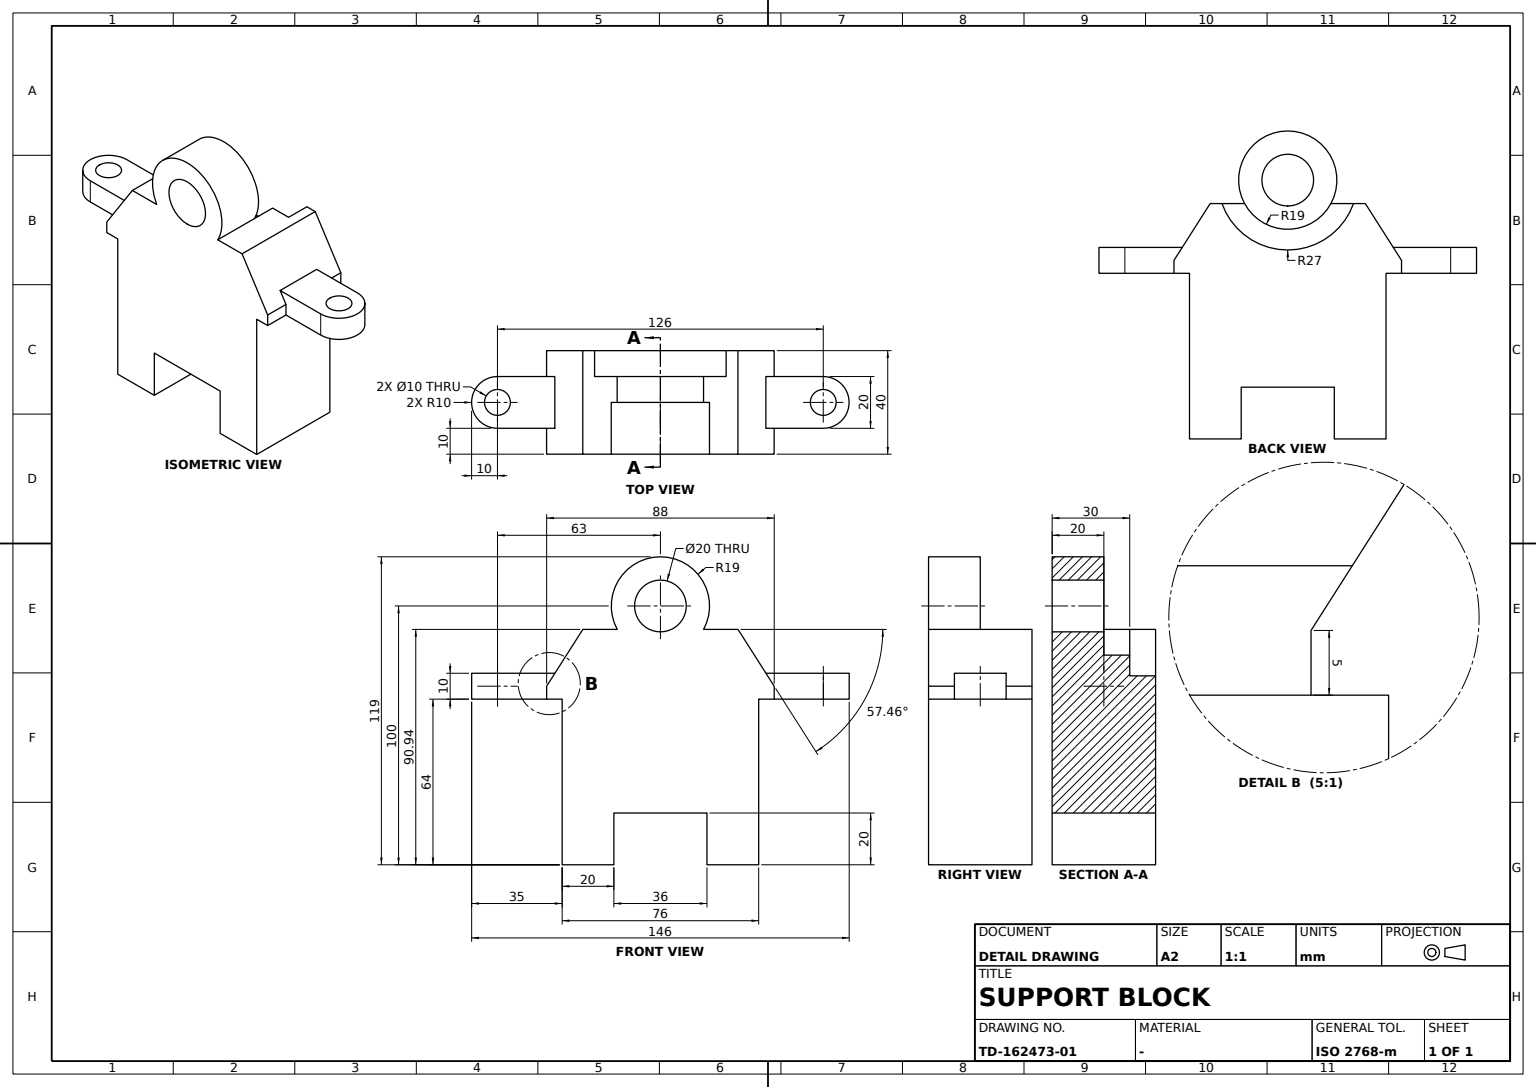
ISO-10303-21;
HEADER;
FILE_DESCRIPTION((''),'2;1');
FILE_NAME('','',(''),(''),'','','');
FILE_SCHEMA(('AUTOMOTIVE_DESIGN'));
ENDSEC;
DATA;
#1=APPLICATION_CONTEXT('');
#2=PRODUCT_CONTEXT('',#1,'mechanical');
#3=PRODUCT('','','',(#2));
#4=PRODUCT_DEFINITION_FORMATION('','',#3);
#5=PRODUCT_DEFINITION_CONTEXT('',#1,'design');
#6=PRODUCT_DEFINITION('','',#4,#5);
#7=PRODUCT_DEFINITION_SHAPE('','',#6);
#8=(LENGTH_UNIT()NAMED_UNIT(*)SI_UNIT(.MILLI.,.METRE.));
#9=(NAMED_UNIT(*)PLANE_ANGLE_UNIT()SI_UNIT($,.RADIAN.));
#10=(NAMED_UNIT(*)SI_UNIT($,.STERADIAN.)SOLID_ANGLE_UNIT());
#11=UNCERTAINTY_MEASURE_WITH_UNIT(LENGTH_MEASURE(0.005),#8,'distance_accuracy_value','');
#12=(GEOMETRIC_REPRESENTATION_CONTEXT(3)GLOBAL_UNCERTAINTY_ASSIGNED_CONTEXT((#11))GLOBAL_UNIT_ASSIGNED_CONTEXT((#8,#9,#10))REPRESENTATION_CONTEXT('',''));
#13=CARTESIAN_POINT('',(44.,10.,64.));
#14=VERTEX_POINT('',#13);
#15=CARTESIAN_POINT('',(44.,20.,64.));
#16=VERTEX_POINT('',#15);
#17=CARTESIAN_POINT('',(44.,0.,64.));
#18=DIRECTION('',(0.,1.,0.));
#19=VECTOR('',#18,1000.);
#20=LINE('',#17,#19);
#21=EDGE_CURVE('',#14,#16,#20,.T.);
#22=ORIENTED_EDGE('',*,*,#21,.T.);
#23=CARTESIAN_POINT('',(44.,20.,69.));
#24=VERTEX_POINT('',#23);
#25=CARTESIAN_POINT('',(44.,20.,0.));
#26=DIRECTION('',(0.,0.,1.));
#27=VECTOR('',#26,1000.);
#28=LINE('',#25,#27);
#29=EDGE_CURVE('',#16,#24,#28,.T.);
#30=ORIENTED_EDGE('',*,*,#29,.T.);
#31=CARTESIAN_POINT('',(44.,10.,69.));
#32=VERTEX_POINT('',#31);
#33=CARTESIAN_POINT('',(44.,0.,69.));
#34=LINE('',#33,#19);
#35=EDGE_CURVE('',#32,#24,#34,.T.);
#36=ORIENTED_EDGE('',*,*,#35,.F.);
#37=LINE('',#13,#27);
#38=EDGE_CURVE('',#14,#32,#37,.T.);
#39=ORIENTED_EDGE('',*,*,#38,.F.);
#40=EDGE_LOOP('',(#22,#30,#36,#39));
#41=FACE_BOUND('',#40,.T.);
#42=DIRECTION('',(-1.,0.,0.));
#43=AXIS2_PLACEMENT_3D('',#17,#42,#26);
#44=PLANE('',#43);
#45=ADVANCED_FACE('',(#41),#44,.F.);
#46=CARTESIAN_POINT('',(-44.,10.,64.));
#47=VERTEX_POINT('',#46);
#48=CARTESIAN_POINT('',(-44.,10.,69.));
#49=VERTEX_POINT('',#48);
#50=CARTESIAN_POINT('',(-44.,10.,0.));
#51=LINE('',#50,#27);
#52=EDGE_CURVE('',#47,#49,#51,.T.);
#53=ORIENTED_EDGE('',*,*,#52,.T.);
#54=CARTESIAN_POINT('',(-44.,20.,69.));
#55=VERTEX_POINT('',#54);
#56=CARTESIAN_POINT('',(-44.,0.,69.));
#57=LINE('',#56,#19);
#58=EDGE_CURVE('',#49,#55,#57,.T.);
#59=ORIENTED_EDGE('',*,*,#58,.T.);
#60=CARTESIAN_POINT('',(-44.,20.,64.));
#61=VERTEX_POINT('',#60);
#62=CARTESIAN_POINT('',(-44.,20.,0.));
#63=DIRECTION('',(0.,0.,-1.));
#64=VECTOR('',#63,1000.);
#65=LINE('',#62,#64);
#66=EDGE_CURVE('',#55,#61,#65,.T.);
#67=ORIENTED_EDGE('',*,*,#66,.T.);
#68=CARTESIAN_POINT('',(-44.,0.,64.));
#69=LINE('',#68,#19);
#70=EDGE_CURVE('',#47,#61,#69,.T.);
#71=ORIENTED_EDGE('',*,*,#70,.F.);
#72=EDGE_LOOP('',(#53,#59,#67,#71));
#73=FACE_BOUND('',#72,.T.);
#74=DIRECTION('',(1.,0.,0.));
#75=AXIS2_PLACEMENT_3D('',#56,#74,#63);
#76=PLANE('',#75);
#77=ADVANCED_FACE('',(#73),#76,.F.);
#78=CARTESIAN_POINT('',(-58.,0.,64.));
#79=VERTEX_POINT('',#78);
#80=CARTESIAN_POINT('',(-63.,0.,64.));
#81=AXIS2_PLACEMENT_3D('',#80,#26,#74);
#82=CIRCLE('',#81,5.);
#83=EDGE_CURVE('',#79,#79,#82,.T.);
#84=ORIENTED_EDGE('',*,*,#83,.F.);
#85=EDGE_LOOP('',(#84));
#86=FACE_BOUND('',#85,.T.);
#87=CARTESIAN_POINT('',(-68.,0.,74.));
#88=VERTEX_POINT('',#87);
#89=CARTESIAN_POINT('',(-63.,0.,74.));
#90=AXIS2_PLACEMENT_3D('',#89,#63,#42);
#91=CIRCLE('',#90,5.);
#92=EDGE_CURVE('',#88,#88,#91,.F.);
#93=ORIENTED_EDGE('',*,*,#92,.T.);
#94=EDGE_LOOP('',(#93));
#95=FACE_BOUND('',#94,.T.);
#96=CARTESIAN_POINT('',(-63.,0.,69.));
#97=AXIS2_PLACEMENT_3D('',#96,#26,#42);
#98=CYLINDRICAL_SURFACE('',#97,5.);
#99=ADVANCED_FACE('',(#86,#95),#98,.F.);
#100=CARTESIAN_POINT('',(-40.81012,10.,74.));
#101=VERTEX_POINT('',#100);
#102=DIRECTION('',(0.537842608,0.,0.843045271));
#103=VECTOR('',#102,1000.);
#104=LINE('',#48,#103);
#105=EDGE_CURVE('',#49,#101,#104,.T.);
#106=ORIENTED_EDGE('',*,*,#105,.F.);
#107=ORIENTED_EDGE('',*,*,#52,.F.);
#108=CARTESIAN_POINT('',(-63.,10.,64.));
#109=VERTEX_POINT('',#108);
#110=VECTOR('',#74,1000.);
#111=LINE('',#46,#110);
#112=EDGE_CURVE('',#109,#47,#111,.T.);
#113=ORIENTED_EDGE('',*,*,#112,.F.);
#114=CARTESIAN_POINT('',(-63.,10.,74.));
#115=VERTEX_POINT('',#114);
#116=CARTESIAN_POINT('',(-63.,10.,69.));
#117=LINE('',#116,#27);
#118=EDGE_CURVE('',#109,#115,#117,.T.);
#119=ORIENTED_EDGE('',*,*,#118,.T.);
#120=CARTESIAN_POINT('',(0.,10.,74.));
#121=LINE('',#120,#110);
#122=EDGE_CURVE('',#115,#101,#121,.T.);
#123=ORIENTED_EDGE('',*,*,#122,.T.);
#124=EDGE_LOOP('',(#106,#107,#113,#119,#123));
#125=FACE_BOUND('',#124,.T.);
#126=CARTESIAN_POINT('',(0.,10.,0.));
#127=DIRECTION('',(0.,-1.,0.));
#128=AXIS2_PLACEMENT_3D('',#126,#127,#74);
#129=PLANE('',#128);
#130=ADVANCED_FACE('',(#125),#129,.F.);
#131=CARTESIAN_POINT('',(-16.703177,-20.,90.944401));
#132=VERTEX_POINT('',#131);
#133=CARTESIAN_POINT('',(-30.,-20.,90.944401));
#134=VERTEX_POINT('',#133);
#135=CARTESIAN_POINT('',(0.,-20.,90.944401));
#136=VECTOR('',#42,1000.);
#137=LINE('',#135,#136);
#138=EDGE_CURVE('',#132,#134,#137,.T.);
#139=ORIENTED_EDGE('',*,*,#138,.T.);
#140=CARTESIAN_POINT('',(-44.,-20.,69.));
#141=VERTEX_POINT('',#140);
#142=CARTESIAN_POINT('',(-62.558286,-20.,39.910682));
#143=LINE('',#142,#103);
#144=EDGE_CURVE('',#141,#134,#143,.T.);
#145=ORIENTED_EDGE('',*,*,#144,.F.);
#146=CARTESIAN_POINT('',(-44.,-20.,64.));
#147=VERTEX_POINT('',#146);
#148=CARTESIAN_POINT('',(-44.,-20.,0.));
#149=LINE('',#148,#64);
#150=EDGE_CURVE('',#141,#147,#149,.T.);
#151=ORIENTED_EDGE('',*,*,#150,.T.);
#152=CARTESIAN_POINT('',(-38.,-20.,64.));
#153=VERTEX_POINT('',#152);
#154=CARTESIAN_POINT('',(0.,-20.,64.));
#155=LINE('',#154,#110);
#156=EDGE_CURVE('',#147,#153,#155,.T.);
#157=ORIENTED_EDGE('',*,*,#156,.T.);
#158=CARTESIAN_POINT('',(-38.,-20.,0.));
#159=VERTEX_POINT('',#158);
#160=LINE('',#158,#27);
#161=EDGE_CURVE('',#159,#153,#160,.T.);
#162=ORIENTED_EDGE('',*,*,#161,.F.);
#163=CARTESIAN_POINT('',(-18.,-20.,0.));
#164=VERTEX_POINT('',#163);
#165=CARTESIAN_POINT('',(0.,-20.,0.));
#166=LINE('',#165,#136);
#167=EDGE_CURVE('',#164,#159,#166,.T.);
#168=ORIENTED_EDGE('',*,*,#167,.F.);
#169=CARTESIAN_POINT('',(-18.,-20.,20.));
#170=VERTEX_POINT('',#169);
#171=LINE('',#163,#64);
#172=EDGE_CURVE('',#170,#164,#171,.T.);
#173=ORIENTED_EDGE('',*,*,#172,.F.);
#174=CARTESIAN_POINT('',(18.,-20.,20.));
#175=VERTEX_POINT('',#174);
#176=CARTESIAN_POINT('',(0.,-20.,20.));
#177=LINE('',#176,#136);
#178=EDGE_CURVE('',#175,#170,#177,.T.);
#179=ORIENTED_EDGE('',*,*,#178,.F.);
#180=CARTESIAN_POINT('',(18.,-20.,0.));
#181=VERTEX_POINT('',#180);
#182=LINE('',#180,#27);
#183=EDGE_CURVE('',#181,#175,#182,.T.);
#184=ORIENTED_EDGE('',*,*,#183,.F.);
#185=CARTESIAN_POINT('',(38.,-20.,0.));
#186=VERTEX_POINT('',#185);
#187=EDGE_CURVE('',#186,#181,#166,.T.);
#188=ORIENTED_EDGE('',*,*,#187,.F.);
#189=CARTESIAN_POINT('',(38.,-20.,64.));
#190=VERTEX_POINT('',#189);
#191=LINE('',#185,#64);
#192=EDGE_CURVE('',#190,#186,#191,.T.);
#193=ORIENTED_EDGE('',*,*,#192,.F.);
#194=CARTESIAN_POINT('',(44.,-20.,64.));
#195=VERTEX_POINT('',#194);
#196=EDGE_CURVE('',#190,#195,#155,.T.);
#197=ORIENTED_EDGE('',*,*,#196,.T.);
#198=CARTESIAN_POINT('',(44.,-20.,69.));
#199=VERTEX_POINT('',#198);
#200=CARTESIAN_POINT('',(44.,-20.,0.));
#201=LINE('',#200,#27);
#202=EDGE_CURVE('',#195,#199,#201,.T.);
#203=ORIENTED_EDGE('',*,*,#202,.T.);
#204=CARTESIAN_POINT('',(30.,-20.,90.944401));
#205=VERTEX_POINT('',#204);
#206=CARTESIAN_POINT('',(62.558286,-20.,39.910682));
#207=DIRECTION('',(-0.537842608,0.,0.843045271));
#208=VECTOR('',#207,1000.);
#209=LINE('',#206,#208);
#210=EDGE_CURVE('',#199,#205,#209,.T.);
#211=ORIENTED_EDGE('',*,*,#210,.T.);
#212=CARTESIAN_POINT('',(16.703177,-20.,90.944401));
#213=VERTEX_POINT('',#212);
#214=EDGE_CURVE('',#205,#213,#137,.T.);
#215=ORIENTED_EDGE('',*,*,#214,.T.);
#216=CARTESIAN_POINT('',(0.,-20.,100.));
#217=AXIS2_PLACEMENT_3D('',#216,#18,#26);
#218=CIRCLE('',#217,19.);
#219=EDGE_CURVE('',#213,#132,#218,.F.);
#220=ORIENTED_EDGE('',*,*,#219,.T.);
#221=EDGE_LOOP('',(#139,#145,#151,#157,#162,#168,#173,#179,#184,#188,#193,#197,#203,#211,#215,#220));
#222=FACE_BOUND('',#221,.T.);
#223=CARTESIAN_POINT('',(0.,-20.,110.));
#224=VERTEX_POINT('',#223);
#225=CIRCLE('',#217,10.);
#226=EDGE_CURVE('',#224,#224,#225,.F.);
#227=ORIENTED_EDGE('',*,*,#226,.F.);
#228=EDGE_LOOP('',(#227));
#229=FACE_BOUND('',#228,.T.);
#230=AXIS2_PLACEMENT_3D('',#165,#18,#42);
#231=PLANE('',#230);
#232=ADVANCED_FACE('',(#222,#229),#231,.F.);
#233=CARTESIAN_POINT('',(-44.,-10.,64.));
#234=VERTEX_POINT('',#233);
#235=CARTESIAN_POINT('',(-63.,-10.,64.));
#236=VERTEX_POINT('',#235);
#237=CARTESIAN_POINT('',(33.,-10.,64.));
#238=LINE('',#237,#136);
#239=EDGE_CURVE('',#234,#236,#238,.T.);
#240=ORIENTED_EDGE('',*,*,#239,.F.);
#241=CARTESIAN_POINT('',(-44.,-10.,69.));
#242=VERTEX_POINT('',#241);
#243=LINE('',#233,#27);
#244=EDGE_CURVE('',#234,#242,#243,.T.);
#245=ORIENTED_EDGE('',*,*,#244,.T.);
#246=CARTESIAN_POINT('',(-40.81012,-10.,74.));
#247=VERTEX_POINT('',#246);
#248=LINE('',#241,#103);
#249=EDGE_CURVE('',#242,#247,#248,.T.);
#250=ORIENTED_EDGE('',*,*,#249,.T.);
#251=CARTESIAN_POINT('',(-63.,-10.,74.));
#252=VERTEX_POINT('',#251);
#253=CARTESIAN_POINT('',(0.,-10.,74.));
#254=LINE('',#253,#136);
#255=EDGE_CURVE('',#247,#252,#254,.T.);
#256=ORIENTED_EDGE('',*,*,#255,.T.);
#257=CARTESIAN_POINT('',(-63.,-10.,69.));
#258=LINE('',#257,#27);
#259=EDGE_CURVE('',#236,#252,#258,.T.);
#260=ORIENTED_EDGE('',*,*,#259,.F.);
#261=EDGE_LOOP('',(#240,#245,#250,#256,#260));
#262=FACE_BOUND('',#261,.T.);
#263=AXIS2_PLACEMENT_3D('',#237,#127,#74);
#264=PLANE('',#263);
#265=ADVANCED_FACE('',(#262),#264,.T.);
#266=ORIENTED_EDGE('',*,*,#219,.F.);
#267=CARTESIAN_POINT('',(16.703177,0.,90.944401));
#268=VERTEX_POINT('',#267);
#269=VECTOR('',#127,1000.);
#270=LINE('',#212,#269);
#271=EDGE_CURVE('',#213,#268,#270,.F.);
#272=ORIENTED_EDGE('',*,*,#271,.T.);
#273=CARTESIAN_POINT('',(-16.703177,0.,90.944401));
#274=VERTEX_POINT('',#273);
#275=CARTESIAN_POINT('',(0.,0.,100.));
#276=AXIS2_PLACEMENT_3D('',#275,#127,#63);
#277=CIRCLE('',#276,19.);
#278=EDGE_CURVE('',#268,#274,#277,.T.);
#279=ORIENTED_EDGE('',*,*,#278,.T.);
#280=LINE('',#131,#269);
#281=EDGE_CURVE('',#132,#274,#280,.F.);
#282=ORIENTED_EDGE('',*,*,#281,.F.);
#283=EDGE_LOOP('',(#266,#272,#279,#282));
#284=FACE_BOUND('',#283,.T.);
#285=CARTESIAN_POINT('',(0.,-10.,100.));
#286=AXIS2_PLACEMENT_3D('',#285,#127,#74);
#287=CYLINDRICAL_SURFACE('',#286,19.);
#288=ADVANCED_FACE('',(#284),#287,.T.);
#289=ORIENTED_EDGE('',*,*,#226,.T.);
#290=EDGE_LOOP('',(#289));
#291=FACE_BOUND('',#290,.T.);
#292=CARTESIAN_POINT('',(0.,0.,90.));
#293=VERTEX_POINT('',#292);
#294=CIRCLE('',#276,10.);
#295=EDGE_CURVE('',#293,#293,#294,.T.);
#296=ORIENTED_EDGE('',*,*,#295,.F.);
#297=EDGE_LOOP('',(#296));
#298=FACE_BOUND('',#297,.T.);
#299=CYLINDRICAL_SURFACE('',#286,10.);
#300=ADVANCED_FACE('',(#291,#298),#299,.F.);
#301=CARTESIAN_POINT('',(58.,0.,74.));
#302=VERTEX_POINT('',#301);
#303=CARTESIAN_POINT('',(63.,0.,74.));
#304=AXIS2_PLACEMENT_3D('',#303,#63,#42);
#305=CIRCLE('',#304,5.);
#306=EDGE_CURVE('',#302,#302,#305,.T.);
#307=ORIENTED_EDGE('',*,*,#306,.F.);
#308=EDGE_LOOP('',(#307));
#309=FACE_BOUND('',#308,.T.);
#310=CARTESIAN_POINT('',(68.,0.,64.));
#311=VERTEX_POINT('',#310);
#312=CARTESIAN_POINT('',(63.,0.,64.));
#313=AXIS2_PLACEMENT_3D('',#312,#26,#74);
#314=CIRCLE('',#313,5.);
#315=EDGE_CURVE('',#311,#311,#314,.F.);
#316=ORIENTED_EDGE('',*,*,#315,.T.);
#317=EDGE_LOOP('',(#316));
#318=FACE_BOUND('',#317,.T.);
#319=CARTESIAN_POINT('',(63.,0.,69.));
#320=AXIS2_PLACEMENT_3D('',#319,#63,#74);
#321=CYLINDRICAL_SURFACE('',#320,5.);
#322=ADVANCED_FACE('',(#309,#318),#321,.F.);
#323=CARTESIAN_POINT('',(38.,20.,0.));
#324=VERTEX_POINT('',#323);
#325=CARTESIAN_POINT('',(38.,0.,0.));
#326=LINE('',#325,#19);
#327=EDGE_CURVE('',#186,#324,#326,.T.);
#328=ORIENTED_EDGE('',*,*,#327,.F.);
#329=ORIENTED_EDGE('',*,*,#187,.T.);
#330=CARTESIAN_POINT('',(18.,20.,0.));
#331=VERTEX_POINT('',#330);
#332=CARTESIAN_POINT('',(18.,0.,0.));
#333=LINE('',#332,#19);
#334=EDGE_CURVE('',#181,#331,#333,.T.);
#335=ORIENTED_EDGE('',*,*,#334,.T.);
#336=CARTESIAN_POINT('',(0.,20.,0.));
#337=LINE('',#336,#136);
#338=EDGE_CURVE('',#324,#331,#337,.T.);
#339=ORIENTED_EDGE('',*,*,#338,.F.);
#340=EDGE_LOOP('',(#328,#329,#335,#339));
#341=FACE_BOUND('',#340,.T.);
#342=AXIS2_PLACEMENT_3D('',#325,#63,#42);
#343=PLANE('',#342);
#344=ADVANCED_FACE('',(#341),#343,.T.);
#345=EDGE_CURVE('',#147,#234,#69,.T.);
#346=ORIENTED_EDGE('',*,*,#345,.F.);
#347=ORIENTED_EDGE('',*,*,#150,.F.);
#348=EDGE_CURVE('',#141,#242,#57,.T.);
#349=ORIENTED_EDGE('',*,*,#348,.T.);
#350=ORIENTED_EDGE('',*,*,#244,.F.);
#351=EDGE_LOOP('',(#346,#347,#349,#350));
#352=FACE_BOUND('',#351,.T.);
#353=ADVANCED_FACE('',(#352),#76,.F.);
#354=CARTESIAN_POINT('',(25.436118,20.,90.944401));
#355=VERTEX_POINT('',#354);
#356=CARTESIAN_POINT('',(-25.436118,20.,90.944401));
#357=VERTEX_POINT('',#356);
#358=CARTESIAN_POINT('',(0.,20.,100.));
#359=AXIS2_PLACEMENT_3D('',#358,#18,#26);
#360=CIRCLE('',#359,27.);
#361=EDGE_CURVE('',#355,#357,#360,.T.);
#362=ORIENTED_EDGE('',*,*,#361,.T.);
#363=CARTESIAN_POINT('',(-25.436118,10.,90.944401));
#364=VERTEX_POINT('',#363);
#365=LINE('',#363,#19);
#366=EDGE_CURVE('',#364,#357,#365,.T.);
#367=ORIENTED_EDGE('',*,*,#366,.F.);
#368=CARTESIAN_POINT('',(25.436118,10.,90.944401));
#369=VERTEX_POINT('',#368);
#370=CARTESIAN_POINT('',(0.,10.,100.));
#371=AXIS2_PLACEMENT_3D('',#370,#127,#63);
#372=CIRCLE('',#371,27.);
#373=EDGE_CURVE('',#364,#369,#372,.T.);
#374=ORIENTED_EDGE('',*,*,#373,.T.);
#375=LINE('',#368,#19);
#376=EDGE_CURVE('',#369,#355,#375,.T.);
#377=ORIENTED_EDGE('',*,*,#376,.T.);
#378=EDGE_LOOP('',(#362,#367,#374,#377));
#379=FACE_BOUND('',#378,.T.);
#380=AXIS2_PLACEMENT_3D('',#275,#18,#42);
#381=CYLINDRICAL_SURFACE('',#380,27.);
#382=ADVANCED_FACE('',(#379),#381,.F.);
#383=CIRCLE('',#81,10.);
#384=EDGE_CURVE('',#109,#236,#383,.T.);
#385=ORIENTED_EDGE('',*,*,#384,.T.);
#386=ORIENTED_EDGE('',*,*,#259,.T.);
#387=CIRCLE('',#90,10.);
#388=EDGE_CURVE('',#115,#252,#387,.F.);
#389=ORIENTED_EDGE('',*,*,#388,.F.);
#390=ORIENTED_EDGE('',*,*,#118,.F.);
#391=EDGE_LOOP('',(#385,#386,#389,#390));
#392=FACE_BOUND('',#391,.T.);
#393=CYLINDRICAL_SURFACE('',#97,10.);
#394=ADVANCED_FACE('',(#392),#393,.T.);
#395=CARTESIAN_POINT('',(-30.,20.,90.944401));
#396=VERTEX_POINT('',#395);
#397=CARTESIAN_POINT('',(0.,20.,90.944401));
#398=LINE('',#397,#136);
#399=EDGE_CURVE('',#357,#396,#398,.T.);
#400=ORIENTED_EDGE('',*,*,#399,.T.);
#401=CARTESIAN_POINT('',(-30.,0.,90.944401));
#402=LINE('',#401,#19);
#403=EDGE_CURVE('',#134,#396,#402,.T.);
#404=ORIENTED_EDGE('',*,*,#403,.F.);
#405=ORIENTED_EDGE('',*,*,#138,.F.);
#406=ORIENTED_EDGE('',*,*,#281,.T.);
#407=CARTESIAN_POINT('',(-16.703177,10.,90.944401));
#408=VERTEX_POINT('',#407);
#409=LINE('',#273,#269);
#410=EDGE_CURVE('',#274,#408,#409,.F.);
#411=ORIENTED_EDGE('',*,*,#410,.T.);
#412=CARTESIAN_POINT('',(0.,10.,90.944401));
#413=LINE('',#412,#110);
#414=EDGE_CURVE('',#364,#408,#413,.T.);
#415=ORIENTED_EDGE('',*,*,#414,.F.);
#416=ORIENTED_EDGE('',*,*,#366,.T.);
#417=EDGE_LOOP('',(#400,#404,#405,#406,#411,#415,#416));
#418=FACE_BOUND('',#417,.T.);
#419=CARTESIAN_POINT('',(-25.436118,0.,90.944401));
#420=AXIS2_PLACEMENT_3D('',#419,#63,#42);
#421=PLANE('',#420);
#422=ADVANCED_FACE('',(#418),#421,.F.);
#423=CARTESIAN_POINT('',(16.703177,10.,90.944401));
#424=VERTEX_POINT('',#423);
#425=CIRCLE('',#371,19.);
#426=EDGE_CURVE('',#408,#424,#425,.T.);
#427=ORIENTED_EDGE('',*,*,#426,.T.);
#428=EDGE_CURVE('',#424,#369,#413,.T.);
#429=ORIENTED_EDGE('',*,*,#428,.T.);
#430=ORIENTED_EDGE('',*,*,#373,.F.);
#431=ORIENTED_EDGE('',*,*,#414,.T.);
#432=EDGE_LOOP('',(#427,#429,#430,#431));
#433=FACE_BOUND('',#432,.T.);
#434=ADVANCED_FACE('',(#433),#129,.F.);
#435=CARTESIAN_POINT('',(18.,20.,20.));
#436=VERTEX_POINT('',#435);
#437=LINE('',#330,#27);
#438=EDGE_CURVE('',#331,#436,#437,.T.);
#439=ORIENTED_EDGE('',*,*,#438,.F.);
#440=ORIENTED_EDGE('',*,*,#334,.F.);
#441=ORIENTED_EDGE('',*,*,#183,.T.);
#442=CARTESIAN_POINT('',(18.,0.,20.));
#443=LINE('',#442,#19);
#444=EDGE_CURVE('',#175,#436,#443,.T.);
#445=ORIENTED_EDGE('',*,*,#444,.T.);
#446=EDGE_LOOP('',(#439,#440,#441,#445));
#447=FACE_BOUND('',#446,.T.);
#448=AXIS2_PLACEMENT_3D('',#332,#42,#26);
#449=PLANE('',#448);
#450=ADVANCED_FACE('',(#447),#449,.T.);
#451=ORIENTED_EDGE('',*,*,#172,.T.);
#452=CARTESIAN_POINT('',(-18.,20.,0.));
#453=VERTEX_POINT('',#452);
#454=CARTESIAN_POINT('',(-18.,0.,0.));
#455=LINE('',#454,#19);
#456=EDGE_CURVE('',#164,#453,#455,.T.);
#457=ORIENTED_EDGE('',*,*,#456,.T.);
#458=CARTESIAN_POINT('',(-18.,20.,20.));
#459=VERTEX_POINT('',#458);
#460=LINE('',#452,#64);
#461=EDGE_CURVE('',#459,#453,#460,.T.);
#462=ORIENTED_EDGE('',*,*,#461,.F.);
#463=CARTESIAN_POINT('',(-18.,0.,20.));
#464=LINE('',#463,#19);
#465=EDGE_CURVE('',#170,#459,#464,.T.);
#466=ORIENTED_EDGE('',*,*,#465,.F.);
#467=EDGE_LOOP('',(#451,#457,#462,#466));
#468=FACE_BOUND('',#467,.T.);
#469=AXIS2_PLACEMENT_3D('',#463,#74,#63);
#470=PLANE('',#469);
#471=ADVANCED_FACE('',(#468),#470,.T.);
#472=ORIENTED_EDGE('',*,*,#426,.F.);
#473=ORIENTED_EDGE('',*,*,#410,.F.);
#474=EDGE_CURVE('',#274,#268,#277,.T.);
#475=ORIENTED_EDGE('',*,*,#474,.T.);
#476=LINE('',#267,#269);
#477=EDGE_CURVE('',#268,#424,#476,.F.);
#478=ORIENTED_EDGE('',*,*,#477,.T.);
#479=EDGE_LOOP('',(#472,#473,#475,#478));
#480=FACE_BOUND('',#479,.T.);
#481=ADVANCED_FACE('',(#480),#287,.F.);
#482=ORIENTED_EDGE('',*,*,#92,.F.);
#483=EDGE_LOOP('',(#482));
#484=FACE_BOUND('',#483,.T.);
#485=ORIENTED_EDGE('',*,*,#388,.T.);
#486=ORIENTED_EDGE('',*,*,#255,.F.);
#487=CARTESIAN_POINT('',(-40.81012,0.,74.));
#488=LINE('',#487,#19);
#489=EDGE_CURVE('',#247,#101,#488,.T.);
#490=ORIENTED_EDGE('',*,*,#489,.T.);
#491=ORIENTED_EDGE('',*,*,#122,.F.);
#492=EDGE_LOOP('',(#485,#486,#490,#491));
#493=FACE_BOUND('',#492,.T.);
#494=CARTESIAN_POINT('',(0.,0.,74.));
#495=AXIS2_PLACEMENT_3D('',#494,#63,#74);
#496=PLANE('',#495);
#497=ADVANCED_FACE('',(#484,#493),#496,.F.);
#498=ORIENTED_EDGE('',*,*,#456,.F.);
#499=ORIENTED_EDGE('',*,*,#167,.T.);
#500=CARTESIAN_POINT('',(-38.,20.,0.));
#501=VERTEX_POINT('',#500);
#502=CARTESIAN_POINT('',(-38.,0.,0.));
#503=LINE('',#502,#19);
#504=EDGE_CURVE('',#159,#501,#503,.T.);
#505=ORIENTED_EDGE('',*,*,#504,.T.);
#506=EDGE_CURVE('',#453,#501,#337,.T.);
#507=ORIENTED_EDGE('',*,*,#506,.F.);
#508=EDGE_LOOP('',(#498,#499,#505,#507));
#509=FACE_BOUND('',#508,.T.);
#510=ADVANCED_FACE('',(#509),#343,.T.);
#511=CARTESIAN_POINT('',(44.,-10.,69.));
#512=VERTEX_POINT('',#511);
#513=CARTESIAN_POINT('',(40.81012,-10.,74.));
#514=VERTEX_POINT('',#513);
#515=LINE('',#511,#208);
#516=EDGE_CURVE('',#512,#514,#515,.T.);
#517=ORIENTED_EDGE('',*,*,#516,.F.);
#518=CARTESIAN_POINT('',(44.,-10.,64.));
#519=VERTEX_POINT('',#518);
#520=LINE('',#518,#27);
#521=EDGE_CURVE('',#519,#512,#520,.T.);
#522=ORIENTED_EDGE('',*,*,#521,.F.);
#523=CARTESIAN_POINT('',(63.,-10.,64.));
#524=VERTEX_POINT('',#523);
#525=LINE('',#233,#110);
#526=EDGE_CURVE('',#519,#524,#525,.T.);
#527=ORIENTED_EDGE('',*,*,#526,.T.);
#528=CARTESIAN_POINT('',(63.,-10.,74.));
#529=VERTEX_POINT('',#528);
#530=CARTESIAN_POINT('',(63.,-10.,69.));
#531=LINE('',#530,#64);
#532=EDGE_CURVE('',#524,#529,#531,.F.);
#533=ORIENTED_EDGE('',*,*,#532,.T.);
#534=CARTESIAN_POINT('',(33.,-10.,74.));
#535=LINE('',#534,#110);
#536=EDGE_CURVE('',#514,#529,#535,.T.);
#537=ORIENTED_EDGE('',*,*,#536,.F.);
#538=EDGE_LOOP('',(#517,#522,#527,#533,#537));
#539=FACE_BOUND('',#538,.T.);
#540=ADVANCED_FACE('',(#539),#264,.T.);
#541=ORIENTED_EDGE('',*,*,#521,.T.);
#542=EDGE_CURVE('',#199,#512,#34,.T.);
#543=ORIENTED_EDGE('',*,*,#542,.F.);
#544=ORIENTED_EDGE('',*,*,#202,.F.);
#545=EDGE_CURVE('',#195,#519,#20,.T.);
#546=ORIENTED_EDGE('',*,*,#545,.T.);
#547=EDGE_LOOP('',(#541,#543,#544,#546));
#548=FACE_BOUND('',#547,.T.);
#549=ADVANCED_FACE('',(#548),#44,.F.);
#550=CARTESIAN_POINT('',(30.,20.,90.944401));
#551=VERTEX_POINT('',#550);
#552=EDGE_CURVE('',#551,#355,#398,.T.);
#553=ORIENTED_EDGE('',*,*,#552,.T.);
#554=ORIENTED_EDGE('',*,*,#376,.F.);
#555=ORIENTED_EDGE('',*,*,#428,.F.);
#556=ORIENTED_EDGE('',*,*,#477,.F.);
#557=ORIENTED_EDGE('',*,*,#271,.F.);
#558=ORIENTED_EDGE('',*,*,#214,.F.);
#559=CARTESIAN_POINT('',(30.,0.,90.944401));
#560=LINE('',#559,#19);
#561=EDGE_CURVE('',#205,#551,#560,.T.);
#562=ORIENTED_EDGE('',*,*,#561,.T.);
#563=EDGE_LOOP('',(#553,#554,#555,#556,#557,#558,#562));
#564=FACE_BOUND('',#563,.T.);
#565=ADVANCED_FACE('',(#564),#421,.F.);
#566=ORIENTED_EDGE('',*,*,#444,.F.);
#567=ORIENTED_EDGE('',*,*,#178,.T.);
#568=ORIENTED_EDGE('',*,*,#465,.T.);
#569=CARTESIAN_POINT('',(0.,20.,20.));
#570=LINE('',#569,#136);
#571=EDGE_CURVE('',#436,#459,#570,.T.);
#572=ORIENTED_EDGE('',*,*,#571,.F.);
#573=EDGE_LOOP('',(#566,#567,#568,#572));
#574=FACE_BOUND('',#573,.T.);
#575=AXIS2_PLACEMENT_3D('',#442,#63,#42);
#576=PLANE('',#575);
#577=ADVANCED_FACE('',(#574),#576,.T.);
#578=CARTESIAN_POINT('',(63.,10.,74.));
#579=VERTEX_POINT('',#578);
#580=CIRCLE('',#304,10.);
#581=EDGE_CURVE('',#579,#529,#580,.T.);
#582=ORIENTED_EDGE('',*,*,#581,.T.);
#583=ORIENTED_EDGE('',*,*,#532,.F.);
#584=CARTESIAN_POINT('',(63.,10.,64.));
#585=VERTEX_POINT('',#584);
#586=CIRCLE('',#313,10.);
#587=EDGE_CURVE('',#585,#524,#586,.F.);
#588=ORIENTED_EDGE('',*,*,#587,.F.);
#589=CARTESIAN_POINT('',(63.,10.,69.));
#590=LINE('',#589,#64);
#591=EDGE_CURVE('',#585,#579,#590,.F.);
#592=ORIENTED_EDGE('',*,*,#591,.T.);
#593=EDGE_LOOP('',(#582,#583,#588,#592));
#594=FACE_BOUND('',#593,.T.);
#595=CYLINDRICAL_SURFACE('',#320,10.);
#596=ADVANCED_FACE('',(#594),#595,.T.);
#597=CARTESIAN_POINT('',(38.,20.,64.));
#598=VERTEX_POINT('',#597);
#599=LINE('',#323,#64);
#600=EDGE_CURVE('',#598,#324,#599,.T.);
#601=ORIENTED_EDGE('',*,*,#600,.F.);
#602=CARTESIAN_POINT('',(38.,0.,64.));
#603=LINE('',#602,#19);
#604=EDGE_CURVE('',#190,#598,#603,.T.);
#605=ORIENTED_EDGE('',*,*,#604,.F.);
#606=ORIENTED_EDGE('',*,*,#192,.T.);
#607=ORIENTED_EDGE('',*,*,#327,.T.);
#608=EDGE_LOOP('',(#601,#605,#606,#607));
#609=FACE_BOUND('',#608,.T.);
#610=AXIS2_PLACEMENT_3D('',#602,#74,#63);
#611=PLANE('',#610);
#612=ADVANCED_FACE('',(#609),#611,.T.);
#613=ORIENTED_EDGE('',*,*,#438,.T.);
#614=ORIENTED_EDGE('',*,*,#571,.T.);
#615=ORIENTED_EDGE('',*,*,#461,.T.);
#616=ORIENTED_EDGE('',*,*,#506,.T.);
#617=CARTESIAN_POINT('',(-38.,20.,64.));
#618=VERTEX_POINT('',#617);
#619=LINE('',#500,#27);
#620=EDGE_CURVE('',#501,#618,#619,.T.);
#621=ORIENTED_EDGE('',*,*,#620,.T.);
#622=CARTESIAN_POINT('',(0.,20.,64.));
#623=LINE('',#622,#110);
#624=EDGE_CURVE('',#61,#618,#623,.T.);
#625=ORIENTED_EDGE('',*,*,#624,.F.);
#626=ORIENTED_EDGE('',*,*,#66,.F.);
#627=CARTESIAN_POINT('',(-62.558286,20.,39.910682));
#628=LINE('',#627,#103);
#629=EDGE_CURVE('',#55,#396,#628,.T.);
#630=ORIENTED_EDGE('',*,*,#629,.T.);
#631=ORIENTED_EDGE('',*,*,#399,.F.);
#632=ORIENTED_EDGE('',*,*,#361,.F.);
#633=ORIENTED_EDGE('',*,*,#552,.F.);
#634=CARTESIAN_POINT('',(62.558286,20.,39.910682));
#635=LINE('',#634,#208);
#636=EDGE_CURVE('',#24,#551,#635,.T.);
#637=ORIENTED_EDGE('',*,*,#636,.F.);
#638=ORIENTED_EDGE('',*,*,#29,.F.);
#639=EDGE_CURVE('',#598,#16,#623,.T.);
#640=ORIENTED_EDGE('',*,*,#639,.F.);
#641=ORIENTED_EDGE('',*,*,#600,.T.);
#642=ORIENTED_EDGE('',*,*,#338,.T.);
#643=EDGE_LOOP('',(#613,#614,#615,#616,#621,#625,#626,#630,#631,#632,#633,#637,#638,#640,#641,#642));
#644=FACE_BOUND('',#643,.T.);
#645=AXIS2_PLACEMENT_3D('',#336,#18,#42);
#646=PLANE('',#645);
#647=ADVANCED_FACE('',(#644),#646,.T.);
#648=CARTESIAN_POINT('',(-38.,0.,64.));
#649=LINE('',#648,#19);
#650=EDGE_CURVE('',#153,#618,#649,.T.);
#651=ORIENTED_EDGE('',*,*,#650,.T.);
#652=ORIENTED_EDGE('',*,*,#620,.F.);
#653=ORIENTED_EDGE('',*,*,#504,.F.);
#654=ORIENTED_EDGE('',*,*,#161,.T.);
#655=EDGE_LOOP('',(#651,#652,#653,#654));
#656=FACE_BOUND('',#655,.T.);
#657=AXIS2_PLACEMENT_3D('',#502,#42,#26);
#658=PLANE('',#657);
#659=ADVANCED_FACE('',(#656),#658,.T.);
#660=ORIENTED_EDGE('',*,*,#210,.F.);
#661=ORIENTED_EDGE('',*,*,#542,.T.);
#662=ORIENTED_EDGE('',*,*,#516,.T.);
#663=CARTESIAN_POINT('',(40.81012,10.,74.));
#664=VERTEX_POINT('',#663);
#665=CARTESIAN_POINT('',(40.81012,0.,74.));
#666=LINE('',#665,#19);
#667=EDGE_CURVE('',#514,#664,#666,.T.);
#668=ORIENTED_EDGE('',*,*,#667,.T.);
#669=LINE('',#31,#208);
#670=EDGE_CURVE('',#32,#664,#669,.T.);
#671=ORIENTED_EDGE('',*,*,#670,.F.);
#672=ORIENTED_EDGE('',*,*,#35,.T.);
#673=ORIENTED_EDGE('',*,*,#636,.T.);
#674=ORIENTED_EDGE('',*,*,#561,.F.);
#675=EDGE_LOOP('',(#660,#661,#662,#668,#671,#672,#673,#674));
#676=FACE_BOUND('',#675,.T.);
#677=DIRECTION('',(-0.843045271,0.,-0.537842608));
#678=AXIS2_PLACEMENT_3D('',#33,#677,#207);
#679=PLANE('',#678);
#680=ADVANCED_FACE('',(#676),#679,.F.);
#681=ORIENTED_EDGE('',*,*,#474,.F.);
#682=ORIENTED_EDGE('',*,*,#278,.F.);
#683=EDGE_LOOP('',(#681,#682));
#684=FACE_BOUND('',#683,.T.);
#685=ORIENTED_EDGE('',*,*,#295,.T.);
#686=EDGE_LOOP('',(#685));
#687=FACE_BOUND('',#686,.T.);
#688=CARTESIAN_POINT('',(0.,0.,0.));
#689=AXIS2_PLACEMENT_3D('',#688,#127,#74);
#690=PLANE('',#689);
#691=ADVANCED_FACE('',(#684,#687),#690,.F.);
#692=ORIENTED_EDGE('',*,*,#639,.T.);
#693=ORIENTED_EDGE('',*,*,#21,.F.);
#694=CARTESIAN_POINT('',(0.,10.,64.));
#695=LINE('',#694,#136);
#696=EDGE_CURVE('',#585,#14,#695,.T.);
#697=ORIENTED_EDGE('',*,*,#696,.F.);
#698=ORIENTED_EDGE('',*,*,#587,.T.);
#699=ORIENTED_EDGE('',*,*,#526,.F.);
#700=ORIENTED_EDGE('',*,*,#545,.F.);
#701=ORIENTED_EDGE('',*,*,#196,.F.);
#702=ORIENTED_EDGE('',*,*,#604,.T.);
#703=EDGE_LOOP('',(#692,#693,#697,#698,#699,#700,#701,#702));
#704=FACE_BOUND('',#703,.T.);
#705=ORIENTED_EDGE('',*,*,#315,.F.);
#706=EDGE_LOOP('',(#705));
#707=FACE_BOUND('',#706,.T.);
#708=AXIS2_PLACEMENT_3D('',#68,#26,#74);
#709=PLANE('',#708);
#710=ADVANCED_FACE('',(#704,#707),#709,.F.);
#711=ORIENTED_EDGE('',*,*,#591,.F.);
#712=ORIENTED_EDGE('',*,*,#696,.T.);
#713=ORIENTED_EDGE('',*,*,#38,.T.);
#714=ORIENTED_EDGE('',*,*,#670,.T.);
#715=LINE('',#120,#136);
#716=EDGE_CURVE('',#579,#664,#715,.T.);
#717=ORIENTED_EDGE('',*,*,#716,.F.);
#718=EDGE_LOOP('',(#711,#712,#713,#714,#717));
#719=FACE_BOUND('',#718,.T.);
#720=ADVANCED_FACE('',(#719),#129,.F.);
#721=ORIENTED_EDGE('',*,*,#144,.T.);
#722=ORIENTED_EDGE('',*,*,#403,.T.);
#723=ORIENTED_EDGE('',*,*,#629,.F.);
#724=ORIENTED_EDGE('',*,*,#58,.F.);
#725=ORIENTED_EDGE('',*,*,#105,.T.);
#726=ORIENTED_EDGE('',*,*,#489,.F.);
#727=ORIENTED_EDGE('',*,*,#249,.F.);
#728=ORIENTED_EDGE('',*,*,#348,.F.);
#729=EDGE_LOOP('',(#721,#722,#723,#724,#725,#726,#727,#728));
#730=FACE_BOUND('',#729,.T.);
#731=DIRECTION('',(-0.843045271,0.,0.537842608));
#732=AXIS2_PLACEMENT_3D('',#56,#731,#102);
#733=PLANE('',#732);
#734=ADVANCED_FACE('',(#730),#733,.T.);
#735=ORIENTED_EDGE('',*,*,#83,.T.);
#736=EDGE_LOOP('',(#735));
#737=FACE_BOUND('',#736,.T.);
#738=ORIENTED_EDGE('',*,*,#239,.T.);
#739=ORIENTED_EDGE('',*,*,#384,.F.);
#740=ORIENTED_EDGE('',*,*,#112,.T.);
#741=ORIENTED_EDGE('',*,*,#70,.T.);
#742=ORIENTED_EDGE('',*,*,#624,.T.);
#743=ORIENTED_EDGE('',*,*,#650,.F.);
#744=ORIENTED_EDGE('',*,*,#156,.F.);
#745=ORIENTED_EDGE('',*,*,#345,.T.);
#746=EDGE_LOOP('',(#738,#739,#740,#741,#742,#743,#744,#745));
#747=FACE_BOUND('',#746,.T.);
#748=ADVANCED_FACE('',(#737,#747),#709,.F.);
#749=ORIENTED_EDGE('',*,*,#306,.T.);
#750=EDGE_LOOP('',(#749));
#751=FACE_BOUND('',#750,.T.);
#752=ORIENTED_EDGE('',*,*,#667,.F.);
#753=ORIENTED_EDGE('',*,*,#536,.T.);
#754=ORIENTED_EDGE('',*,*,#581,.F.);
#755=ORIENTED_EDGE('',*,*,#716,.T.);
#756=EDGE_LOOP('',(#752,#753,#754,#755));
#757=FACE_BOUND('',#756,.T.);
#758=ADVANCED_FACE('',(#751,#757),#496,.F.);
#759=CLOSED_SHELL('',(#45,#77,#99,#130,#232,#265,#288,#300,#322,#344,#353,#382,#394,#422,#434,#450,#471,#481,#497,#510,#540,#549,#565,#577,#596,#612,#647,#659,#680,#691,#710,#720,#734,#748,#758));
#760=MANIFOLD_SOLID_BREP('',#759);
#761=ADVANCED_BREP_SHAPE_REPRESENTATION('',(#760),#12);
#762=SHAPE_DEFINITION_REPRESENTATION(#7,#761);
ENDSEC;
END-ISO-10303-21;
